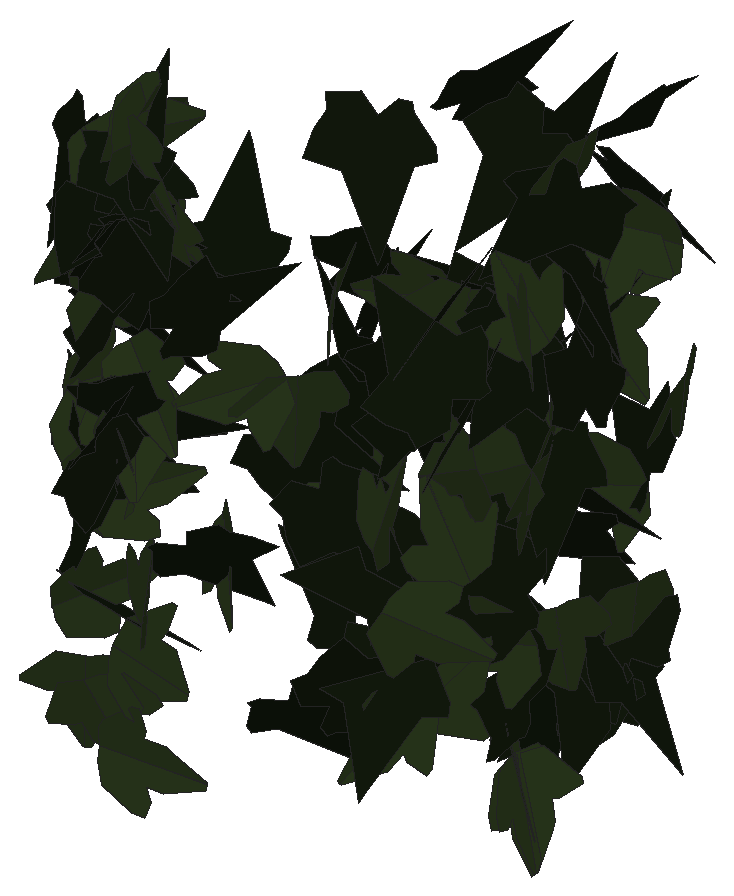
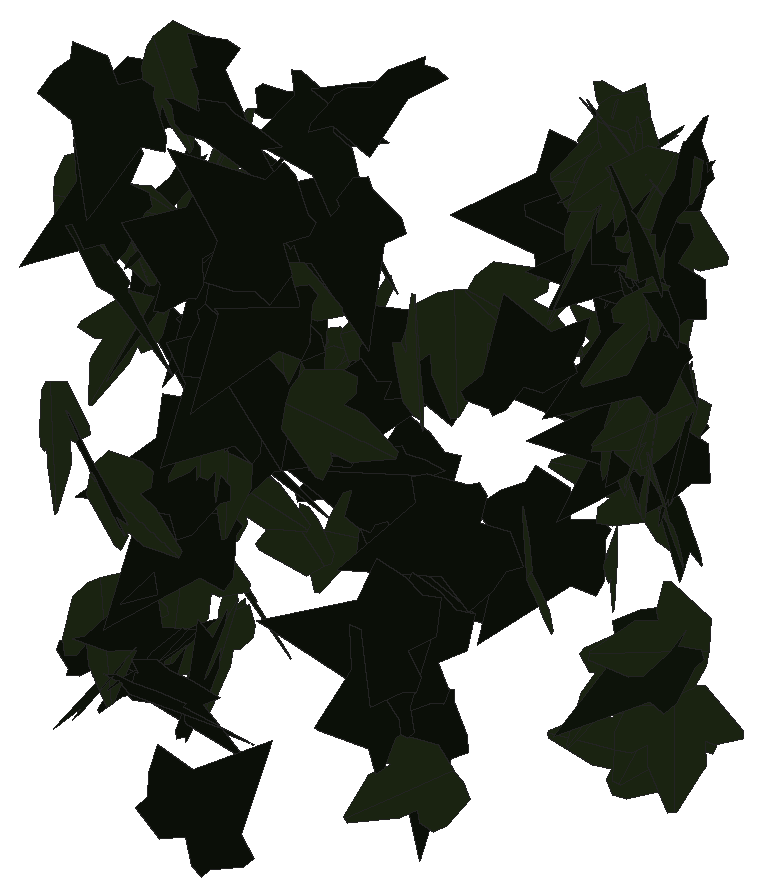
# SketchUp Ruby script. Lengths in inches.
U = 1.inch
M = Sketchup.active_model
def pt(a) = Geom::Point3d.new(a.map { |v| v * U })
def face(e, loops, mat)
  f = e.add_face(loops[0].map { |a| pt(a) })
  loops[1..].each { |l| e.add_face(l.map { |a| pt(a) }).erase! }
  f.material = f.back_material = mat if mat
  f
end
# faces: each face lists its corners as indices into pts; further lists are holes
def faces(e, pts, list, mat = nil) = list.each { |f| face(e, (f[0].is_a?(Array) ? f : [f]).map { |l| l.map { |i| pts[i] } }, mat) }
# xy, xz, yz: faces in a plane at the given z, y or x. An outline is a flat list of corners, or four numbers for a rectangle; further outlines are holes
def ring(l) = l.size == 4 ? [[l[0], l[1]], [l[2], l[1]], [l[2], l[3]], [l[0], l[3]]] : l.each_slice(2).to_a
def flat(e, list, mat, &to3) = list.each { |f| face(e, (f[0].is_a?(Array) ? f : [f]).map { |l| ring(l).map { |u, v| to3.(u, v) } }, mat) }
def xy(e, z, list, mat = nil) = flat(e, list, mat) { |x, y| [x, y, z] }
def xz(e, y, list, mat = nil) = flat(e, list, mat) { |x, z| [x, y, z] }
def yz(e, x, list, mat = nil) = flat(e, list, mat) { |y, z| [x, y, z] }
def lines(e, pts, list) = list.each { |a, b| e.add_line(pt(pts[a]), pt(pts[b])) }
# prism: a flat outline (further loops are holes) pulled along v
def prism(e, loops, v, mat = nil)
  f = face(e, loops, mat); d = Geom::Vector3d.new(v.map { |x| x * U })
  f.pushpull(f.normal.samedirection?(d) ? d.length : -d.length)
end
def box(e, o, s, mat = nil) = prism(e, [[o, [o[0] + s[0], o[1], o[2]], [o[0] + s[0], o[1] + s[1], o[2]], [o[0], o[1] + s[1], o[2]]]], [0, 0, s[2]], mat)
def at(x, y, z, deg = 0) = Geom::Transformation.translation(pt([x, y, z])) * Geom::Transformation.rotation(ORIGIN, Z_AXIS, deg.degrees)
def axes(o, x, y, z) = Geom::Transformation.new([*x, 0, *y, 0, *z, 0, *pt(o).to_a, 1])
def part(name) = M.definitions.add(name)
# library, detail: a bought-in or finely detailed component or shape, given as its bounding box
def library(name, o, s) = part(name).tap { |d| box(d.entities, o, s) }
def detail(e, o, s) = box(e.add_group.entities, o, s)
def put(e, d, t, mat = nil) = e.add_instance(d, t).tap { |i| i.material = mat if mat }
def group(e, t, mat = nil) = e.add_group.tap { |g| g.transformation = t; g.material = mat if mat }.entities
root = M.entities
M.materials.add("efeu1").color = [18, 25, 13]
M.materials.add("efeu2").color = [43, 57, 29]
c1 = part("ivyleaf_10")
p = [[0,0.5,-0.03],[-0.0625,2.02,-0.43],[-0.19,2.01,-0.46],[-0.54,1.05,-0.29],[-0.52,0.625,-0.18],[-0.83,0.76,-0.28],
  [-1.16,0.64,-0.33],[-1.15,0.33,-0.24],[-0.77,-0.39,0.02],[-0.3,-0.51,0.16],[0.04,-0.48,0.23],[-0.02,2.01,-0.4375],
  [-0.06,2.01,-0.43],[0.04,-0.49,0.23],[0.67,-0.49,0.14],[1.38,0.36,-0.2],[1.375,0.51,-0.24],[0.81,0.65,-0.19],
  [0.62,0.59,-0.15],[0.6,1.09,-0.28],[0.5,1.23,-0.31]]
faces(c1.entities,p,[[0,1,2,3,4,5,6,7,8,9,10],[11,12,0,13,14,15,16,17,18,19,20]],"efeu2")
c2 = part("ivyleaf_9")
p = [[1.54,2.16,1.25],[1.36,2.04,1.19],[-0.21,0.99,0.68],[-0.71,1.11,0.82],[-0.85,0.86,0.67],[-0.8,0.17,0.21],
  [-0.9,-0.01,0.1],[-0.67,-0.16,-0.02],[-0.08,-0.08,-0.05],[-0.03,-0.6,-0.4],[0.65,-0.88,-0.66],[0.83,-0.6,-0.49],
  [1.29,-0.42,-0.43],[1.8125,-0.07,-0.26],[1.21,0.44,0.15]]
faces(c2.entities,p,[[0,1,2,3,4,5,6,7,8,9,10,11,12,13,14]],"efeu1")
put(root,c1,axes([46.61,221.88,207.375],[-0.41581,-0.27532,0.03602],[-0.03032,-0.01945,-0.4987],[0.27601,-0.41692,-0.00052]))
put(root,c2,axes([46.375,222.11,213.55],[0.04571,-0.01994,-0.49751],[0.38008,-0.32133,0.0478],[-0.32163,-0.38256,-0.01422]))
put(root,c2,axes([46.82,222.15,212.94],[-0.05884,0.23649,0.43659],[-0.09828,0.4254,-0.24368],[-0.4867,-0.11449,-0.00357]))
put(root,c2,axes([46.63,226.41,209.49],[0.06564,0.1606,0.46893],[0.11419,0.45541,-0.17195],[-0.48234,0.12967,0.02311]))
put(root,c1,axes([46.45,221.92,208.13],[0.03415,-0.14531,0.4772],[0.11559,0.4676,0.13411],[-0.48526,0.10116,0.06553]))
put(root,c2,axes([46.45,222.12,210.06],[-0.04948,-0.06044,0.49386],[0.03855,-0.49527,-0.05675],[0.49605,0.03246,0.05367]))
put(root,c1,axes([46.625,221.85,210.77],[0.01302,0.01311,0.49966],[-0.00294,0.49982,-0.01304],[-0.49982,-0.00259,0.0131]))
put(root,c2,axes([46.47,222.05,208.21],[0.49827,-0.02263,-0.03485],[-0.02504,0.1712,-0.46911],[0.03316,0.46923,0.16947]))
put(root,c1,axes([46.74,221.74,212.6],[-0.13473,-0.46175,-0.13653],[0.05434,0.12629,-0.48073],[0.47843,-0.14437,0.01615]))
put(root,c1,axes([46.65,221.94,209.37],[0.45188,-0.21393,0.00622],[-0.00557,0.00278,0.49996],[-0.21395,-0.45191,0.00013]))
put(root,c1,axes([46.48,225.8125,208.39],[0.2016,0.15045,0.43211],[0.31841,0.29297,-0.25056],[-0.32859,0.37621,0.02232]))
put(root,c1,axes([46.66,221.96,213.48],[0.18512,0.41401,0.21054],[0.06113,0.20296,-0.45285],[-0.46043,0.1934,0.02453]))
put(root,c1,axes([46.73,221.52,210.23],[0.06729,0.11578,-0.48173],[0.15523,0.45675,0.13146],[0.47051,-0.16725,0.02552]))
put(root,c1,axes([47,221.79,210.56],[-0.32409,0.22531,0.30693],[-0.25539,0.1703,-0.39468],[-0.28239,-0.4126,0.0047]))
put(root,c2,axes([47.07,221.36,209.44],[-0.10471,0.32375,0.36637],[-0.10773,0.35018,-0.34024],[-0.4769,-0.15019,-0.00358]))
put(root,c1,axes([46.6875,221.98,211.86],[-0.08936,-0.26386,-0.4152],[0.2467,0.34106,-0.26984],[0.42562,-0.25309,0.06924]))
put(root,c2,axes([46.46,226.33,210.09],[0.27135,-0.03634,0.41839],[0.41995,0.01966,-0.27066],[0.00322,0.49829,0.04119]))
put(root,c2,axes([46.78,221.72,213.09],[0.15591,-0.34836,-0.32301],[-0.1323,0.29468,-0.38166],[0.45628,0.20448,-0.00029]))
put(root,c2,axes([46.64,222.07,211.67],[0.49224,0.03043,0.08229],[0.08177,0.01072,-0.49315],[-0.03178,0.49896,0.00558]))
put(root,c2,axes([47.21,221.53,211.87],[-0.24973,0.40427,0.15557],[-0.08293,0.13163,-0.47518],[-0.42515,-0.26314,0.00131]))
put(root,c2,axes([47.15,225.75,209.16],[0.0925,-0.16437,0.46306],[-0.22747,0.40334,0.18861],[-0.43555,-0.24556,-0.00016]))
put(root,c2,axes([47.1,221.8,212.85],[-0.13617,0.46368,-0.12828],[0.03637,-0.12302,-0.48326],[-0.47972,-0.14094,-0.00023]))
put(root,c1,axes([46.8125,222.06,210.73],[-0.18014,0.3707,-0.28307],[0.10536,-0.26327,-0.41181],[-0.45437,-0.20802,0.01673]))
put(root,c1,axes([47.02,222.2,213.51],[0.06433,-0.03702,0.49446],[-0.18337,0.46148,0.05841],[-0.46069,-0.18885,0.04579]))
put(root,c1,axes([46.93,221.63,207.32],[-0.43903,-0.16182,-0.17626],[0.16605,0.05913,-0.4679],[0.17227,-0.46938,0.00183]))
put(root,c2,axes([46.68,221.76,210.49],[0.11225,0.19976,-0.4444],[0.22395,0.38387,0.22911],[0.43272,-0.25048,-0.00329]))
put(root,c2,axes([46.68,221.8,212.36],[0.13187,0.17465,-0.44956],[0.24656,0.37615,0.21845],[0.41451,-0.2793,0.01308]))
put(root,c2,axes([47.15,221.37,210.56],[0.06591,0.37619,0.32271],[0.05631,0.31776,-0.38192],[-0.49243,0.08669,-0.00048]))
put(root,c1,axes([47.05,222.11,210.67],[0.0559,-0.48131,0.12334],[0.16325,-0.09944,-0.46202],[0.46928,0.09192,0.14603]))
put(root,c1,axes([47.02,221.99,213.83],[-0.04314,-0.10448,-0.48705],[0.21644,0.43639,-0.11278],[0.44866,-0.22057,0.00758]))
put(root,c2,axes([47.23,221.77,213.34],[-0.39969,0.29879,0.03117],[0.02277,-0.02159,0.49901],[0.29955,0.40032,0.00365]))
put(root,c1,axes([47.14,221.8,213.78],[0.00866,-0.10688,-0.48837],[0.08626,0.48143,-0.10384],[0.49243,-0.08246,0.02677]))
put(root,c2,axes([47.21,223.47,211.57],[-0.24883,-0.24713,0.35639],[0.27267,0.23036,0.35012],[-0.33724,0.36859,0.02013]))
put(root,c2,axes([47.09,221.59,212.59],[0.23942,0.33895,0.27891],[0.16731,0.22325,-0.41493],[-0.40581,0.29201,-0.00652]))
put(root,c2,axes([47.15,221.41,210.32],[0.00979,-0.02686,-0.49918],[-0.11815,0.48501,-0.02841],[0.48574,0.11852,0.00315]))
put(root,c1,axes([47.19,221.87,207.75],[-0.02911,0.33921,0.36618],[-0.02734,0.36517,-0.34045],[-0.4984,-0.03984,-0.00272]))
put(root,c1,axes([47.22,221.87,210.71],[0.38268,0.32081,0.02519],[0.01938,0.01609,-0.49937],[-0.32121,0.38317,-0.00011]))
put(root,c1,axes([47.09,221.63,209.67],[-0.09287,-0.13645,0.47197],[0.25051,0.40004,0.16495],[-0.42263,0.26711,-0.00594]))
put(root,c2,axes([47.06,222.09,213.45],[0.05625,-0.49462,0.04675],[0.16134,-0.02631,-0.47252],[0.4699,0.06824,0.15664]))
put(root,c1,axes([47.3,222.1875,212.68],[0.11308,-0.37687,-0.30852],[0.13895,0.32853,-0.35038],[0.4668,-0.0065,0.17903]))
put(root,c1,axes([47.18,221.92,213.69],[-0.22399,0.18165,-0.40845],[0.33361,-0.23616,-0.28798],[-0.29754,-0.40154,-0.0154]))
put(root,c2,axes([47.09,221.61,210.64],[0.29994,0.04819,0.39713],[0.39324,0.05564,-0.30376],[-0.07347,0.49455,-0.00453]))
put(root,c2,axes([47.12,225.03,209.15],[0.16069,0.04042,0.47175],[0.46619,0.07355,-0.1651],[-0.08274,0.49291,-0.01405]))
put(root,c1,axes([47.15,221.72,206.64],[0.01054,-0.02201,0.4994],[0.46592,0.18144,-0.00184],[-0.18114,0.4654,0.02434]))
put(root,c1,axes([47.23,221.89,211.19],[0.37213,0.03693,0.33189],[0.33102,0.02478,-0.37391],[-0.04407,0.49802,-0.006]))
put(root,c1,axes([47.3125,222.12,212.84],[0.44655,-0.05984,0.21682],[0.2248,0.10248,-0.4347],[0.00759,0.48571,0.11843]))
put(root,c1,axes([47.71,221.35,208.73],[-0.00909,0.1067,-0.4884],[-0.14769,0.4661,0.10458],[0.4776,0.14616,0.02304]))
put(root,c2,axes([47.18,221.51,212.58],[0.18268,0.08988,-0.45667],[0.30909,0.34336,0.19123],[0.34798,-0.35217,0.06989]))
put(root,c2,axes([47.6875,224.39,208.09],[0.32338,0.10039,-0.3679],[-0.36664,-0.05082,-0.33614],[-0.10488,0.48718,0.04074]))
put(root,c2,axes([47.8,222.08,209.16],[0.39818,0.30034,0.03527],[0.02689,0.02292,-0.49875],[-0.30121,0.39908,0.0021]))
put(root,c1,axes([47.65,222.75,208.93],[0.24832,-0.13969,0.41088],[0.36289,-0.19278,-0.28486],[0.238,0.43968,0.00564]))
put(root,c2,axes([47.76,223.5625,209.8125],[0.05266,0.05132,-0.49456],[0.23122,0.43776,0.07004],[0.44019,-0.23608,0.02237]))
put(root,c1,axes([48.17,223.99,211.32],[0.12096,-0.3124,-0.37118],[0.1393,-0.34407,0.33498],[-0.46472,-0.18444,0.0038]))
put(root,c1,axes([48.6875,222.11,211.39],[0.23689,0.03803,-0.43868],[-0.43658,-0.04448,-0.23961],[-0.05725,0.49656,0.01213]))
put(root,c2,axes([48.21,221.37,212.22],[0.1203,0.1168,0.47105],[0.35889,0.30527,-0.16735],[-0.32669,0.37838,-0.01039]))
put(root,c1,axes([48.84,224.78,211.24],[0.10277,0.03722,-0.48791],[-0.48549,0.07008,-0.09691],[0.06118,0.49366,0.05054]))
put(root,c2,axes([49.14,223.05,208.46],[-0.12797,0.13193,0.46499],[-0.32707,0.33053,-0.18379],[-0.35588,-0.35121,0.0017]))
put(root,c1,axes([48.93,222.41,211.24],[-0.30296,-0.39776,0.00217],[-0.00073,-0.00217,-0.49999],[0.39776,-0.30296,0.00074]))
put(root,c2,axes([48.86,225.27,213.38],[0.19634,0.45466,-0.06879],[0.01254,0.06948,0.49499],[0.45967,-0.1961,0.01588]))
put(root,c2,axes([49.5,225.87,206.75],[0.20966,-0.11102,0.44013],[-0.39116,0.20178,0.23723],[-0.2303,-0.4438,-0.00224]))
put(root,c2,axes([49.23,223.34,214.1],[-0.08281,-0.48281,-0.10021],[0.01735,0.09869,-0.48986],[0.49279,-0.08461,0.00041]))
put(root,c2,axes([49.39,221.75,208.04],[0.34977,0.35729,-0.00259],[-0.00377,0.00006,-0.49999],[-0.35728,0.34978,0.00274]))
put(root,c1,axes([49.92,224,211.91],[-0.452,-0.1955,0.08645],[-0.06697,-0.06253,-0.49153],[0.20301,-0.45593,0.03034]))
put(root,c2,axes([49.83,225.3,212.875],[-0.03226,-0.04398,0.49702],[0.27678,0.41282,0.0545],[-0.41515,0.27865,-0.00229]))
put(root,c2,axes([49.79,224.12,211.97],[0.4672,0.16086,-0.07647],[-0.10016,0.05975,-0.48621],[-0.14728,0.46963,0.08806]))
put(root,c2,axes([49.63,221.97,210.48],[-0.0511,-0.10014,-0.4872],[0.32395,0.36493,-0.10899],[0.37742,-0.3268,0.02758]))
put(root,c2,axes([50.1,224.09,211.5],[0.06168,0.45819,-0.19043],[-0.06071,-0.18348,-0.46114],[-0.49245,0.08,0.033]))
put(root,c2,axes([50.18,224.3125,210.83],[0.16051,0.33461,0.33507],[0.05384,0.3386,-0.36394],[-0.47047,0.15291,0.07266]))
put(root,c2,axes([50.43,222.45,209.51],[-0.16063,-0.08808,0.46523],[-0.40212,-0.23401,-0.18314],[0.25,-0.43299,0.00434]))
put(root,c2,axes([50.36,222.47,212.02],[0.24401,0.24204,-0.36315],[-0.26734,-0.24595,-0.34356],[-0.34494,0.36184,0.00939]))
put(root,c2,axes([50.03,224.24,211.52],[-0.23975,0.06028,0.43461],[0.42134,-0.10656,0.24722],[0.12243,0.48478,0.0003]))
put(root,c2,axes([50.09,224.06,210.24],[-0.04681,-0.36672,-0.33664],[0.02865,0.33558,-0.36954],[0.49698,-0.05389,-0.0104]))
put(root,c1,axes([50.29,224.2,210.22],[-0.02305,-0.47779,-0.14554],[0.02217,0.14457,-0.47813],[0.49898,-0.0285,0.01452]))
put(root,c2,axes([50.46,224.43,213.86],[-0.48275,-0.11675,-0.05767],[0.05615,0.01316,-0.49666],[0.11749,-0.486,0.00041]))
put(root,c1,axes([50.4,221.85,210.37],[0.00877,0.20126,-0.45762],[-0.04514,0.45614,0.19975],[0.49788,0.03781,0.02617]))
put(root,c2,axes([50.1,221.56,208.37],[0.10326,0.01455,0.489],[0.45194,0.18851,-0.10105],[-0.1873,0.46287,0.02578]))
put(root,c1,axes([50.36,224.37,210.38],[-0.00277,0.4882,-0.10796],[-0.02697,-0.10795,-0.48746],[-0.49926,0.00312,0.02693]))
put(root,c2,axes([50.32,224.16,212.12],[0.11575,-0.29123,-0.3896],[-0.1536,0.3581,-0.31332],[0.46153,0.19222,-0.00656]))
put(root,c2,axes([50.66,222.81,211.5],[-0.12413,0.48218,-0.04573],[0.01202,-0.04413,-0.4979],[-0.4842,-0.12471,-0.00064]))
put(root,c1,axes([50.56,222.18,208.15],[0.12085,0.24194,-0.42055],[-0.18194,-0.37917,-0.27042],[-0.44977,0.21839,-0.00361]))
put(root,c2,axes([50.52,222.01,208.78],[-0.26492,-0.41737,-0.07495],[0.04205,0.06208,-0.49435],[0.42196,-0.26823,0.00221]))
put(root,c2,axes([50.94,221.87,211.89],[-0.30502,0.35047,0.18475],[-0.12324,0.13766,-0.46461],[-0.37653,-0.32897,0.00241]))
put(root,c2,axes([50.83,224.92,207.62],[-0.49007,-0.09814,0.01418],[-0.01261,-0.00924,-0.49976],[0.09835,-0.49019,0.00658]))
put(root,c2,axes([50.5625,224.41,209.29],[0.35525,0.33309,0.11335],[0.05334,0.10824,-0.48522],[-0.34778,0.35684,0.04137]))
put(root,c2,axes([50.76,222.08,212.53],[-0.20909,0.37221,-0.26028],[-0.14697,0.21567,0.42648],[0.42975,0.25485,0.01921]))
put(root,c2,axes([50.99,225.02,207.51],[-0.49101,0.00728,0.09411],[-0.09287,-0.12639,-0.47476],[0.01688,-0.48371,0.12547]))
put(root,c2,axes([50.86,224.01,206.97],[-0.0146,-0.27736,0.41576],[0.0946,0.40689,0.27476],[-0.49075,0.08668,0.0406]))
put(root,c1,axes([51.09,225.1,209.72],[0.18415,-0.07278,-0.45912],[-0.42926,0.1629,-0.19799],[0.1784,0.46708,-0.00249]))
put(root,c2,axes([50.41,224.46,209.94],[0.4384,-0.07904,0.22706],[0.22902,-0.00637,-0.44442],[0.07315,0.49367,0.03062]))
put(root,c1,axes([51.16,222.43,211.1],[-0.22489,0.0473,0.44406],[-0.44431,0.02625,-0.22781],[-0.04486,-0.49707,0.03022]))
put(root,c1,axes([50.91,222.57,209.89],[0.08331,0.48139,0.10639],[-0.02278,-0.10403,0.48853],[0.49248,-0.08624,0.0046]))
put(root,c2,axes([50.75,224.53,212.23],[0.39592,-0.1586,-0.26095],[-0.2277,0.13136,-0.42532],[0.20347,0.45562,0.03179]))
put(root,c1,axes([50.59,222.65,208.18],[0.37251,-0.09971,-0.31827],[0.30887,-0.0769,0.38559],[-0.12584,-0.48389,0.0043]))
put(root,c2,axes([51.17,225.28,212.47],[-0.37581,0.32737,0.03996],[-0.03282,0.02316,-0.49838],[-0.32816,-0.37722,0.00408]))
put(root,c1,axes([51.02,223.95,210.91],[0.19822,-0.42659,-0.16949],[-0.07047,0.15415,-0.47039],[0.45359,0.21037,0.00099]))
put(root,c1,axes([50.97,224.11,208.5],[-0.27449,-0.40877,-0.08698],[0.05403,0.06848,-0.49233],[0.41441,-0.27968,0.00658]))
put(root,c2,axes([51.13,225.08,207.78],[-0.35664,-0.31684,0.14975],[0.12651,0.08285,0.47658],[-0.32681,0.37782,0.02107]))
put(root,c1,axes([51.32,222.96,208.86],[0.1412,0.01395,-0.47945],[-0.46804,0.11329,-0.13455],[0.10488,0.4868,0.04505]))
put(root,c2,axes([51.32,223.16,208.125],[-0.31128,0.31932,0.22613],[-0.15501,0.16469,-0.44593],[-0.35927,-0.34772,-0.00353]))
put(root,c2,axes([51.31,225.18,209.95],[-0.12098,0.2179,0.43345],[-0.20604,0.38136,-0.24922],[-0.43922,-0.23892,-0.00248]))
put(root,c1,axes([51.35,222.92,210.99],[-0.24012,-0.04359,0.4364],[-0.42639,-0.09325,-0.24392],[0.10265,-0.48929,0.00761]))
put(root,c2,axes([50.9,224.83,207.67],[-0.07158,-0.47756,0.12966],[-0.00744,-0.12996,-0.48276],[0.49479,-0.07104,0.0115]))
put(root,c2,axes([51.4,223.01,209.46],[-0.41962,0.19125,0.19323],[-0.17817,0.07498,-0.46112],[-0.20536,-0.45585,0.00522]))
put(root,c2,axes([51.16,224.95,214.13],[0.10484,0.47519,0.11489],[-0.03843,0.12515,-0.48256],[-0.48737,0.09235,0.06276]))
put(root,c1,axes([50.97,224.82,211.59],[0.0558,0.43199,0.24551],[0.02819,0.2439,-0.43557],[-0.49608,0.06245,0.00287]))
put(root,c1,axes([51.12,223.5625,212.3],[-0.01053,0.46831,0.17485],[-0.00068,-0.17491,0.46841],[0.49989,0.00962,0.00431]))
put(root,c2,axes([51.38,221.81,212.33],[-0.44627,-0.20649,-0.0906],[-0.08197,-0.0386,0.49172],[-0.21007,0.45373,0.0006]))
put(root,c2,axes([51.17,222.66,212.09],[-0.34149,0.25763,-0.25886],[0.20815,-0.15391,-0.42777],[-0.30009,-0.39992,-0.00214]))
put(root,c2,axes([50.81,225.24,213.3],[0.49207,-0.08227,0.0331],[0.03335,-0.00129,-0.49889],[0.08217,0.49318,0.00422]))
put(root,c1,axes([51.16,225.13,208.41],[-0.13568,-0.48094,-0.01707],[0.00729,0.01568,-0.4997],[0.48118,-0.13585,0.00275]))
put(root,c2,axes([51.03,223.4,212.03],[-0.07131,-0.40527,0.28402],[-0.03718,-0.28176,-0.41138],[0.49349,-0.07979,0.01005]))
put(root,c2,axes([50.82,224.52,212.74],[0.24931,-0.408,0.14622],[0.08642,-0.1185,-0.47801],[0.42471,0.26362,0.01144]))
put(root,c1,axes([51.1,223.28,207.46],[-0.2518,0.42888,-0.05155],[0.02319,-0.04616,-0.49732],[-0.43134,-0.25285,0.00335]))
put(root,c1,axes([51.16,224.89,212.83],[0.46918,0.13872,-0.10308],[-0.10054,-0.02347,-0.48922],[-0.14057,0.4798,0.00587]))
put(root,c1,axes([51.23,224.1,214.0625],[0.068,-0.4886,0.0815],[0.00094,-0.08213,-0.49321],[0.49535,0.06723,-0.01025]))
put(root,c1,axes([51.57,225,212.81],[-0.0101,0.02053,-0.49948],[-0.49951,0.01929,0.01089],[0.01972,0.49921,0.02012]))
put(root,c1,axes([50.98,221.61,209.64],[-0.20218,-0.1498,-0.43207],[0.38598,0.19744,-0.24907],[0.24524,-0.43425,0.0358]))
put(root,c2,axes([51.44,223.86,213.82],[0.03258,0.15866,-0.47304],[-0.12525,-0.45627,-0.16166],[-0.48296,0.12903,0.01002]))
put(root,c2,axes([50.99,225.04,207.8],[0.2801,-0.40554,-0.08415],[-0.00664,0.09718,-0.49042],[0.41413,0.27585,0.04906]))
put(root,c1,axes([51.37,225.64,210.77],[0.09673,-0.4419,-0.21299],[-0.05464,0.20604,-0.45229],[0.4875,0.11077,-0.00843]))
put(root,c1,axes([51.49,222.95,212.36],[-0.07747,0.21469,-0.44487],[-0.19474,0.40056,0.22722],[0.45395,0.20848,0.02155]))
put(root,c2,axes([51.24,223.7,210.9],[-0.34781,-0.2092,-0.292],[0.24984,0.15113,-0.40588],[0.25808,-0.42825,-0.0006]))
put(root,c2,axes([51.41,224.03,211.28],[-0.12394,-0.25004,0.41487],[0.17357,0.37688,0.27899],[-0.45223,0.21318,-0.00662]))
put(root,c1,axes([51.28,223.16,207.2],[-0.0007,0.49989,-0.01063],[0.00211,-0.01063,-0.49988],[-0.5,-0.00074,-0.00209]))
put(root,c1,axes([51.28,223.18,207.18],[0.09315,0.49124,0.0028],[0.00141,0.00258,-0.49999],[-0.49124,0.09316,-0.00091]))
put(root,c1,axes([51.43,223.25,210.81],[0.16594,-0.47153,0.01103],[0.0037,-0.0104,-0.49988],[0.47165,0.16598,0.00004]))
